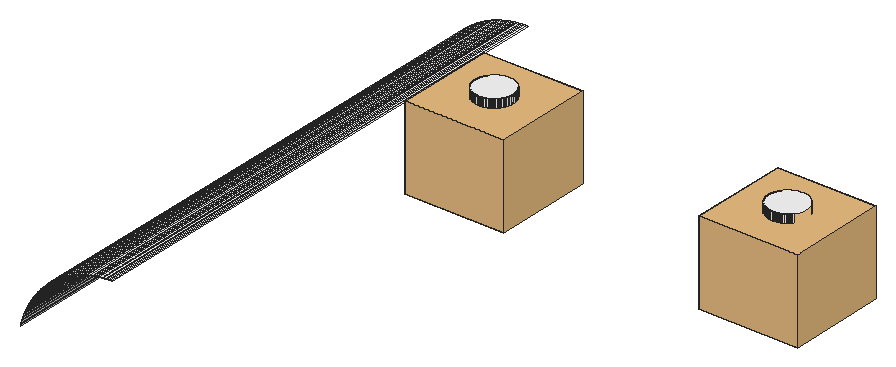
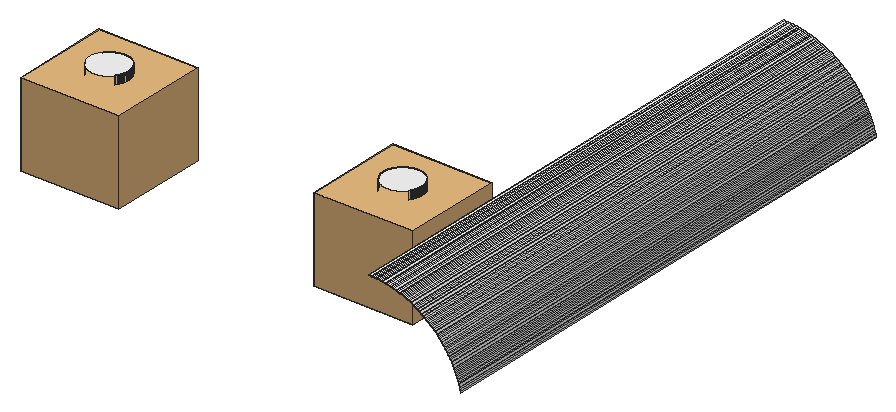
# SketchUp Ruby script. Lengths in inches.
U = 1.inch
M = Sketchup.active_model
def pt(a) = Geom::Point3d.new(a.map { |v| v * U })
def face(e, loops, mat)
  f = e.add_face(loops[0].map { |a| pt(a) })
  loops[1..].each { |l| e.add_face(l.map { |a| pt(a) }).erase! }
  f.material = f.back_material = mat if mat
  f
end
# faces: each face lists its corners as indices into pts; further lists are holes
def faces(e, pts, list, mat = nil) = list.each { |f| face(e, (f[0].is_a?(Array) ? f : [f]).map { |l| l.map { |i| pts[i] } }, mat) }
# xy, xz, yz: faces in a plane at the given z, y or x. An outline is a flat list of corners, or four numbers for a rectangle; further outlines are holes
def ring(l) = l.size == 4 ? [[l[0], l[1]], [l[2], l[1]], [l[2], l[3]], [l[0], l[3]]] : l.each_slice(2).to_a
def flat(e, list, mat, &to3) = list.each { |f| face(e, (f[0].is_a?(Array) ? f : [f]).map { |l| ring(l).map { |u, v| to3.(u, v) } }, mat) }
def xy(e, z, list, mat = nil) = flat(e, list, mat) { |x, y| [x, y, z] }
def xz(e, y, list, mat = nil) = flat(e, list, mat) { |x, z| [x, y, z] }
def yz(e, x, list, mat = nil) = flat(e, list, mat) { |y, z| [x, y, z] }
def lines(e, pts, list) = list.each { |a, b| e.add_line(pt(pts[a]), pt(pts[b])) }
# prism: a flat outline (further loops are holes) pulled along v
def prism(e, loops, v, mat = nil)
  f = face(e, loops, mat); d = Geom::Vector3d.new(v.map { |x| x * U })
  f.pushpull(f.normal.samedirection?(d) ? d.length : -d.length)
end
def box(e, o, s, mat = nil) = prism(e, [[o, [o[0] + s[0], o[1], o[2]], [o[0] + s[0], o[1] + s[1], o[2]], [o[0], o[1] + s[1], o[2]]]], [0, 0, s[2]], mat)
def at(x, y, z, deg = 0) = Geom::Transformation.translation(pt([x, y, z])) * Geom::Transformation.rotation(ORIGIN, Z_AXIS, deg.degrees)
def axes(o, x, y, z) = Geom::Transformation.new([*x, 0, *y, 0, *z, 0, *pt(o).to_a, 1])
def part(name) = M.definitions.add(name)
# library, detail: a bought-in or finely detailed component or shape, given as its bounding box
def library(name, o, s) = part(name).tap { |d| box(d.entities, o, s) }
def detail(e, o, s) = box(e.add_group.entities, o, s)
def put(e, d, t, mat = nil) = e.add_instance(d, t).tap { |i| i.material = mat if mat }
def group(e, t, mat = nil) = e.add_group.tap { |g| g.transformation = t; g.material = mat if mat }.entities
root = M.entities
M.materials.add("[Quartz Light Grey]").color = [251, 251, 252]
c1 = library("5",[-6.25,-6.25,-13.16],[15.58,15.58,13.16])
xy(root,116.99,[[59.41,189,59.61,271]],"[Quartz Light Grey]")
xy(root,117,[[59.8,189,60,271]],"[Quartz Light Grey]")
xy(root,119.5,[[68.84,250,68.76,250.01,68.6875,250.02,68.61,250.03,68.45,250.05,68.375,250.07,68.3,250.08,68.22,250.1,68.15,250.125,68.07,250.15,68,250.17,67.92,250.2,67.71,250.29,67.64,250.33,67.57,250.36,67.43,250.44,67.37,250.48,67.3,250.53,67.24,250.57,67.17,250.62,66.93,250.82,66.88,250.88,66.82,250.93,66.62,251.17,66.57,251.24,66.53,251.3,66.48,251.37,66.44,251.43,66.36,251.57,66.33,251.64,66.29,251.71,66.2,251.92,66.17,252,66.15,252.07,66.125,252.15,66.1,252.22,66.08,252.3,66.07,252.375,66.05,252.45,66.03,252.61,66.02,252.6875,66.01,252.76,66,252.84,66,253.16,66.01,253.24,66.02,253.3125,66.03,253.39,66.05,253.55,66.07,253.625,66.08,253.7,66.1,253.78,66.125,253.85,66.15,253.93,66.17,254,66.2,254.08,66.29,254.29,66.33,254.36,66.36,254.43,66.44,254.57,66.48,254.63,66.53,254.7,66.57,254.76,66.62,254.83,66.82,255.07,66.88,255.12,66.93,255.18,67.17,255.38,67.24,255.43,67.3,255.47,67.37,255.52,67.43,255.56,67.57,255.64,67.64,255.67,67.71,255.71,67.92,255.8,68,255.83,68.07,255.85,68.15,255.875,68.22,255.9,68.3,255.92,68.375,255.93,68.45,255.95,68.61,255.97,68.6875,255.98,68.76,255.99,68.84,256,69.16,256,69.24,255.99,69.3125,255.98,69.39,255.97,69.55,255.95,69.625,255.93,69.7,255.92,69.78,255.9,69.85,255.875,69.93,255.85,70,255.83,70.08,255.8,70.29,255.71,70.36,255.67,70.43,255.64,70.57,255.56,70.63,255.52,70.7,255.47,70.76,255.43,70.83,255.38,71.07,255.18,71.12,255.12,71.18,255.07,71.38,254.83,71.43,254.76,71.47,254.7,71.52,254.63,71.56,254.57,71.64,254.43,71.67,254.36,71.71,254.29,71.8,254.08,71.83,254,71.85,253.93,71.875,253.85,71.9,253.78,71.92,253.7,71.93,253.625,71.95,253.55,71.97,253.39,71.98,253.3125,71.99,253.24,72,253.16,72,252.84,71.99,252.76,71.98,252.6875,71.97,252.61,71.95,252.45,71.93,252.375,71.92,252.3,71.9,252.22,71.875,252.15,71.85,252.07,71.83,252,71.8,251.92,71.71,251.71,71.67,251.64,71.64,251.57,71.56,251.43,71.52,251.37,71.47,251.3,71.43,251.24,71.38,251.17,71.18,250.93,71.12,250.88,71.07,250.82,70.83,250.62,70.76,250.57,70.7,250.53,70.63,250.48,70.57,250.44,70.43,250.36,70.36,250.33,70.29,250.29,70.08,250.2,70,250.17,69.93,250.15,69.85,250.125,69.78,250.1,69.7,250.08,69.625,250.07,69.55,250.05,69.39,250.03,69.3125,250.02,69.24,250.01,69.16,250],[115.18,250,114.86,250.04,114.79,250.05,114.71,250.07,114.63,250.08,114.56,250.1,114.48,250.125,114.41,250.15,114.33,250.17,114.19,250.23,114.11,250.26,114.04,250.29,113.97,250.33,113.9,250.36,113.83,250.4,113.77,250.44,113.7,250.48,113.63,250.53,113.57,250.57,113.45,250.67,113.38,250.72,113.33,250.77,113.27,250.82,113.1,250.99,112.95,251.17,112.91,251.24,112.86,251.3,112.82,251.37,112.78,251.43,112.66,251.64,112.59,251.78,112.5625,251.85,112.53,251.92,112.51,252,112.48,252.07,112.46,252.15,112.4375,252.22,112.42,252.3,112.38,252.45,112.36,252.61,112.35,252.6875,112.34,252.76,112.34,252.84,112.33,252.92,112.33,253.08,112.34,253.16,112.34,253.24,112.35,253.3125,112.36,253.39,112.38,253.55,112.42,253.7,112.4375,253.78,112.46,253.85,112.48,253.93,112.51,254,112.53,254.08,112.5625,254.15,112.59,254.22,112.66,254.36,112.78,254.57,112.82,254.63,112.86,254.7,112.91,254.76,112.95,254.83,113.1,255.01,113.27,255.18,113.33,255.23,113.38,255.28,113.45,255.33,113.57,255.43,113.63,255.47,113.7,255.52,113.77,255.56,113.83,255.6,113.9,255.64,113.97,255.67,114.04,255.71,114.11,255.74,114.19,255.77,114.33,255.83,114.41,255.85,114.48,255.875,114.56,255.9,114.63,255.92,114.71,255.93,114.79,255.95,114.86,255.96,115.18,256,115.49,256,115.65,255.98,115.72,255.97,115.88,255.95,115.96,255.93,116.03,255.92,116.11,255.9,116.19,255.875,116.26,255.85,116.33,255.83,116.41,255.8,116.55,255.74,116.625,255.71,116.7,255.67,116.76,255.64,116.97,255.52,117.03,255.47,117.1,255.43,117.4,255.18,117.45,255.12,117.51,255.07,117.5625,255.01,117.61,254.95,117.71,254.83,117.76,254.76,117.81,254.7,117.85,254.63,117.89,254.57,118.01,254.36,118.13,254.08,118.16,254,118.1875,253.93,118.21,253.85,118.23,253.78,118.25,253.7,118.27,253.625,118.28,253.55,118.3,253.47,118.31,253.39,118.32,253.3125,118.32,253.24,118.33,253.16,118.33,252.84,118.32,252.76,118.32,252.6875,118.31,252.61,118.3,252.53,118.28,252.45,118.27,252.375,118.25,252.3,118.23,252.22,118.21,252.15,118.1875,252.07,118.16,252,118.13,251.92,118.01,251.64,117.89,251.43,117.85,251.37,117.81,251.3,117.76,251.24,117.71,251.17,117.61,251.05,117.5625,250.99,117.51,250.93,117.45,250.88,117.4,250.82,117.1,250.57,117.03,250.53,116.97,250.48,116.76,250.36,116.7,250.33,116.625,250.29,116.55,250.26,116.41,250.2,116.33,250.17,116.26,250.15,116.19,250.125,116.11,250.1,116.03,250.08,115.96,250.07,115.88,250.05,115.72,250.03,115.65,250.02,115.49,250]],"[Quartz Light Grey]")
xz(root,250,[[68.84,117,68.92,119.5],[68.92,117,69,119.5],[69,117,69.08,119.5],[69.08,117,69.16,119.5],[115.18,117,115.25,119.5],
  [115.25,117,115.33,119.5],[115.33,117,115.41,119.5],[115.41,117,115.49,119.5]],"[Quartz Light Grey]")
yz(root,66,[[252.84,117,252.92,119.5],[252.92,117,253,119.5],[253,117,253.08,119.5],[253.08,117,253.16,119.5]],"[Quartz Light Grey]")
yz(root,72,[[252.84,117,252.92,119.5],[252.92,117,253,119.5],[253,117,253.08,119.5],[253.08,117,253.16,119.5]],"[Quartz Light Grey]")
yz(root,112.33,[[252.92,117,253,119.5],[253,117,253.08,119.5]],"[Quartz Light Grey]")
yz(root,112.34,[[252.76,117,252.84,119.5],[253.16,117,253.24,119.5]],"[Quartz Light Grey]")
p = [[45.46,271,105.69],[45.46,189,105.69],[45.41,189,105.5],[45.41,271,105.5],[45.51,271,105.88],[45.51,189,105.88],
  [45.5625,271,106.07],[45.5625,189,106.07],[45.62,271,106.26],[45.62,189,106.26],[45.67,271,106.45],[45.67,189,106.45],
  [45.73,271,106.64],[45.73,189,106.64],[45.8,271,106.82],[45.8,189,106.82],[45.86,271,107.01],[45.86,189,107.01],
  [45.93,271,107.19],[45.93,189,107.19],[46,271,107.375],[46,189,107.375],[46.07,271,107.56],[46.07,189,107.56],
  [46.14,271,107.74],[46.14,189,107.74],[46.22,271,107.92],[46.22,189,107.92],[46.3,271,108.1],[46.3,189,108.1],
  [46.38,271,108.28],[46.38,189,108.28],[46.46,271,108.46],[46.46,189,108.46],[46.55,271,108.63],[46.55,189,108.63],
  [46.63,271,108.81],[46.63,189,108.81],[46.73,271,108.98],[46.73,189,108.98],[46.82,271,109.16],[46.82,189,109.16],
  [46.91,271,109.33],[46.91,189,109.33],[47.01,271,109.5],[47.01,189,109.5],[47.11,271,109.67],[47.11,189,109.67],
  [47.21,271,109.84],[47.21,189,109.84],[47.3125,271,110],[47.3125,189,110],[47.42,271,110.17],[47.42,189,110.17],
  [47.53,271,110.33],[47.53,189,110.33],[47.64,271,110.5],[47.64,189,110.5],[47.75,271,110.66],[47.75,189,110.66],
  [47.86,271,110.82],[47.86,189,110.82],[47.98,271,110.97],[47.98,189,110.97],[48.1,271,111.13],[48.1,189,111.13],
  [48.22,271,111.29],[48.22,189,111.29],[48.34,271,111.44],[48.34,189,111.44],[48.47,271,111.59],[48.47,189,111.59],
  [48.59,271,111.74],[48.59,189,111.74],[48.72,271,111.89],[48.72,189,111.89],[48.85,271,112.04],[48.85,189,112.04],
  [48.99,271,112.18],[48.99,189,112.18],[49.12,271,112.33],[49.12,189,112.33],[49.26,271,112.47],[49.26,189,112.47],
  [49.39,271,112.61],[49.39,189,112.61],[49.53,271,112.74],[49.53,189,112.74],[49.67,271,112.88],[49.67,189,112.88],
  [49.82,271,113.01],[49.82,189,113.01],[49.96,271,113.15],[49.96,189,113.15],[50.11,271,113.28],[50.11,189,113.28],
  [50.26,271,113.41],[50.26,189,113.41],[50.41,271,113.53],[50.41,189,113.53],[50.56,271,113.66],[50.56,189,113.66],
  [50.71,271,113.78],[50.71,189,113.78],[50.87,271,113.9],[50.87,189,113.9],[51.03,271,114.02],[51.03,189,114.02],
  [51.18,271,114.14],[51.18,189,114.14],[51.34,271,114.25],[51.34,189,114.25],[51.5,271,114.36],[51.5,189,114.36],
  [51.67,271,114.47],[51.67,189,114.47],[51.83,271,114.58],[51.83,189,114.58],[52,271,114.6875],[52,189,114.6875],
  [52.16,271,114.79],[52.16,189,114.79],[52.33,271,114.89],[52.33,189,114.89],[52.5,271,114.99],[52.5,189,114.99],
  [52.67,271,115.09],[52.67,189,115.09],[52.84,271,115.18],[52.84,189,115.18],[53.02,271,115.27],[53.02,189,115.27],
  [53.19,271,115.37],[53.19,189,115.37],[53.37,271,115.45],[53.37,189,115.45],[53.54,271,115.54],[53.54,189,115.54],
  [53.72,271,115.62],[53.72,189,115.62],[53.9,271,115.7],[53.9,189,115.7],[54.08,271,115.78],[54.08,189,115.78],
  [54.26,271,115.86],[54.26,189,115.86],[54.44,271,115.93],[54.44,189,115.93],[54.625,271,116],[54.625,189,116],
  [54.81,271,116.07],[54.81,189,116.07],[54.99,271,116.14],[54.99,189,116.14],[55.18,271,116.2],[55.18,189,116.2],
  [55.36,271,116.27],[55.36,189,116.27],[55.55,271,116.33],[55.55,189,116.33],[55.74,271,116.38],[55.74,189,116.38],
  [55.93,271,116.4375],[55.93,189,116.4375],[56.12,271,116.49],[56.12,189,116.49],[56.31,271,116.54],[56.31,189,116.54],
  [56.5,271,116.59],[56.5,189,116.59],[56.69,271,116.63],[56.69,189,116.63],[56.88,271,116.67],[56.88,189,116.67],
  [57.07,271,116.71],[57.07,189,116.71],[57.27,271,116.75],[57.27,189,116.75],[57.46,271,116.78],[57.46,189,116.78],
  [57.65,271,116.82],[57.65,189,116.82],[57.85,271,116.84],[57.85,189,116.84],[58.04,271,116.87],[58.04,189,116.87],
  [58.24,271,116.9],[58.24,189,116.9],[58.43,271,116.92],[58.43,189,116.92],[58.63,271,116.9375],[58.63,189,116.9375],
  [58.82,271,116.95],[58.82,189,116.95],[59.02,271,116.97],[59.02,189,116.97],[59.21,271,116.98],[59.21,189,116.98],
  [59.41,271,116.99],[59.41,189,116.99],[59.8,271,117],[59.8,189,117],[59.61,189,116.99],[59.61,271,116.99],
  [68.53,250.04,117],[68.45,250.05,117],[68.45,250.05,119.5],[68.53,250.04,119.5],[68.61,250.03,117],[68.61,250.03,119.5],
  [68.6875,250.02,117],[68.6875,250.02,119.5],[68.76,250.01,117],[68.76,250.01,119.5],[68.84,250,117],[68.84,250,119.5],
  [69.24,250.01,117],[69.16,250,117],[69.16,250,119.5],[69.24,250.01,119.5],[69.3125,250.02,117],[69.3125,250.02,119.5],
  [69.39,250.03,117],[69.39,250.03,119.5],[69.47,250.04,117],[69.47,250.04,119.5],[69.55,250.05,117],[69.55,250.05,119.5],
  [114.86,250.04,117],[114.79,250.05,117],[114.79,250.05,119.5],[114.86,250.04,119.5],[114.94,250.03,117],[114.94,250.03,119.5],
  [115.02,250.02,117],[115.02,250.02,119.5],[115.1,250.01,117],[115.1,250.01,119.5],[115.18,250,117],[115.18,250,119.5],
  [115.57,250.01,117],[115.49,250,117],[115.49,250,119.5],[115.57,250.01,119.5],[115.65,250.02,117],[115.65,250.02,119.5],
  [115.72,250.03,117],[115.72,250.03,119.5],[115.8,250.04,117],[115.8,250.04,119.5],[115.88,250.05,117],[115.88,250.05,119.5],
  [68.07,250.15,117],[68,250.17,117],[68,250.17,119.5],[68.07,250.15,119.5],[68.15,250.125,117],[68.15,250.125,119.5],
  [68.22,250.1,117],[68.22,250.1,119.5],[68.3,250.08,117],[68.3,250.08,119.5],[68.375,250.07,117],[68.375,250.07,119.5],
  [69.625,250.07,117],[69.625,250.07,119.5],[69.7,250.08,117],[69.7,250.08,119.5],[69.78,250.1,117],[69.78,250.1,119.5],
  [69.85,250.125,117],[69.85,250.125,119.5],[69.93,250.15,117],[69.93,250.15,119.5],[70,250.17,117],[70,250.17,119.5],
  [114.41,250.15,117],[114.33,250.17,117],[114.33,250.17,119.5],[114.41,250.15,119.5],[114.48,250.125,117],[114.48,250.125,119.5],
  [114.56,250.1,117],[114.56,250.1,119.5],[114.63,250.08,117],[114.63,250.08,119.5],[114.71,250.07,117],[114.71,250.07,119.5],
  [115.96,250.07,117],[115.96,250.07,119.5],[116.03,250.08,117],[116.03,250.08,119.5],[116.11,250.1,117],[116.11,250.1,119.5],
  [116.19,250.125,117],[116.19,250.125,119.5],[116.26,250.15,117],[116.26,250.15,119.5],[116.33,250.17,117],[116.33,250.17,119.5],
  [67.85,250.23,117],[67.78,250.26,117],[67.78,250.26,119.5],[67.85,250.23,119.5],[67.92,250.2,117],[67.92,250.2,119.5],
  [70.08,250.2,117],[70.08,250.2,119.5],[70.15,250.23,117],[70.15,250.23,119.5],[70.22,250.26,117],[70.22,250.26,119.5],
  [114.19,250.23,117],[114.11,250.26,117],[114.11,250.26,119.5],[114.19,250.23,119.5],[114.26,250.2,117],[114.26,250.2,119.5],
  [116.41,250.2,117],[116.41,250.2,119.5],[116.48,250.23,117],[116.48,250.23,119.5],[116.55,250.26,117],[116.55,250.26,119.5],
  [67.64,250.33,117],[67.57,250.36,117],[67.57,250.36,119.5],[67.64,250.33,119.5],[67.71,250.29,117],[67.71,250.29,119.5],
  [70.29,250.29,117],[70.29,250.29,119.5],[70.36,250.33,117],[70.36,250.33,119.5],[70.43,250.36,117],[70.43,250.36,119.5],
  [113.97,250.33,117],[113.9,250.36,117],[113.9,250.36,119.5],[113.97,250.33,119.5],[114.04,250.29,117],[114.04,250.29,119.5],
  [116.625,250.29,117],[116.625,250.29,119.5],[116.7,250.33,117],[116.7,250.33,119.5],[116.76,250.36,117],[116.76,250.36,119.5],
  [67.43,250.44,117],[67.37,250.48,117],[67.37,250.48,119.5],[67.43,250.44,119.5],[67.5,250.4,117],[67.5,250.4,119.5],
  [70.5,250.4,117],[70.5,250.4,119.5],[70.57,250.44,117],[70.57,250.44,119.5],[70.63,250.48,117],[70.63,250.48,119.5],
  [113.77,250.44,117],[113.7,250.48,117],[113.7,250.48,119.5],[113.77,250.44,119.5],[113.83,250.4,117],[113.83,250.4,119.5],
  [116.83,250.4,117],[116.83,250.4,119.5],[116.9,250.44,117],[116.9,250.44,119.5],[116.97,250.48,117],[116.97,250.48,119.5],
  [67.3,250.53,117],[67.24,250.57,117],[67.24,250.57,119.5],[67.3,250.53,119.5],[70.7,250.53,117],[70.7,250.53,119.5],
  [70.76,250.57,117],[70.76,250.57,119.5],[113.63,250.53,117],[113.57,250.57,117],[113.57,250.57,119.5],[113.63,250.53,119.5],
  [117.03,250.53,117],[117.03,250.53,119.5],[117.1,250.57,117],[117.1,250.57,119.5],[67.17,250.62,117],[67.11,250.67,117],
  [67.11,250.67,119.5],[67.17,250.62,119.5],[70.83,250.62,117],[70.83,250.62,119.5],[70.89,250.67,117],[70.89,250.67,119.5],
  [113.51,250.62,117],[113.45,250.67,117],[113.45,250.67,119.5],[113.51,250.62,119.5],[117.16,250.62,117],[117.16,250.62,119.5],
  [117.22,250.67,117],[117.22,250.67,119.5],[67.05,250.72,117],[66.99,250.77,117],[66.99,250.77,119.5],[67.05,250.72,119.5],
  [70.95,250.72,117],[70.95,250.72,119.5],[71.01,250.77,117],[71.01,250.77,119.5],[113.38,250.72,117],[113.33,250.77,117],
  [113.33,250.77,119.5],[113.38,250.72,119.5],[117.28,250.72,117],[117.28,250.72,119.5],[117.34,250.77,117],[117.34,250.77,119.5],
  [66.93,250.82,117],[66.88,250.88,117],[66.88,250.88,119.5],[66.93,250.82,119.5],[71.07,250.82,117],[71.07,250.82,119.5],
  [71.12,250.88,117],[71.12,250.88,119.5],[113.27,250.82,117],[113.21,250.88,117],[113.21,250.88,119.5],[113.27,250.82,119.5],
  [117.4,250.82,117],[117.4,250.82,119.5],[117.45,250.88,117],[117.45,250.88,119.5],[66.82,250.93,117],[66.77,250.99,117],
  [66.77,250.99,119.5],[66.82,250.93,119.5],[71.18,250.93,117],[71.18,250.93,119.5],[71.23,250.99,117],[71.23,250.99,119.5],
  [113.16,250.93,117],[113.1,250.99,117],[113.1,250.99,119.5],[113.16,250.93,119.5],[117.51,250.93,117],[117.51,250.93,119.5],
  [117.5625,250.99,117],[117.5625,250.99,119.5],[66.72,251.05,117],[66.72,251.05,119.5],[71.28,251.05,117],[71.28,251.05,119.5],
  [113.05,251.05,117],[113.05,251.05,119.5],[117.61,251.05,117],[117.61,251.05,119.5],[66.67,251.11,117],[66.62,251.17,117],
  [66.62,251.17,119.5],[66.67,251.11,119.5],[71.33,251.11,117],[71.33,251.11,119.5],[71.38,251.17,117],[71.38,251.17,119.5],
  [113,251.11,117],[112.95,251.17,117],[112.95,251.17,119.5],[113,251.11,119.5],[117.66,251.11,117],[117.66,251.11,119.5],
  [117.71,251.17,117],[117.71,251.17,119.5],[66.57,251.24,117],[66.53,251.3,117],[66.53,251.3,119.5],[66.57,251.24,119.5],
  [71.43,251.24,117],[71.43,251.24,119.5],[71.47,251.3,117],[71.47,251.3,119.5],[112.91,251.24,117],[112.86,251.3,117],
  [112.86,251.3,119.5],[112.91,251.24,119.5],[117.76,251.24,117],[117.76,251.24,119.5],[66.48,251.37,117],[66.48,251.37,119.5],
  [71.52,251.37,117],[71.52,251.37,119.5],[112.82,251.37,117],[112.82,251.37,119.5],[66.44,251.43,117],[66.4,251.5,117],
  [66.4,251.5,119.5],[66.44,251.43,119.5],[71.56,251.43,117],[71.56,251.43,119.5],[71.6,251.5,117],[71.6,251.5,119.5],
  [112.78,251.43,117],[112.74,251.5,117],[112.74,251.5,119.5],[112.78,251.43,119.5],[66.36,251.57,117],[66.36,251.57,119.5],
  [71.64,251.57,117],[71.64,251.57,119.5],[112.7,251.57,117],[112.7,251.57,119.5],[66.33,251.64,117],[66.29,251.71,117],
  [66.29,251.71,119.5],[66.33,251.64,119.5],[71.67,251.64,117],[71.67,251.64,119.5],[71.71,251.71,117],[71.71,251.71,119.5],
  [112.66,251.64,117],[112.625,251.71,117],[112.625,251.71,119.5],[112.66,251.64,119.5],[66.26,251.78,117],[66.26,251.78,119.5],
  [71.74,251.78,117],[71.74,251.78,119.5],[112.59,251.78,117],[112.59,251.78,119.5],[66.23,251.85,117],[66.23,251.85,119.5],
  [71.77,251.85,117],[71.77,251.85,119.5],[112.5625,251.85,117],[112.5625,251.85,119.5],[66.2,251.92,117],[66.17,252,117],
  [66.17,252,119.5],[66.2,251.92,119.5],[71.8,251.92,117],[71.8,251.92,119.5],[71.83,252,117],[71.83,252,119.5],
  [112.53,251.92,117],[112.51,252,117],[112.51,252,119.5],[112.53,251.92,119.5],[66.15,252.07,117],[66.15,252.07,119.5],
  [71.85,252.07,117],[71.85,252.07,119.5],[112.48,252.07,117],[112.48,252.07,119.5],[66.125,252.15,117],[66.1,252.22,117],
  [66.1,252.22,119.5],[66.125,252.15,119.5],[71.875,252.15,117],[71.875,252.15,119.5],[71.9,252.22,117],[71.9,252.22,119.5],
  [112.46,252.15,117],[112.4375,252.22,117],[112.4375,252.22,119.5],[112.46,252.15,119.5],[66.08,252.3,117],[66.08,252.3,119.5],
  [71.92,252.3,117],[71.92,252.3,119.5],[112.42,252.3,117],[112.42,252.3,119.5],[66.07,252.375,117],[66.07,252.375,119.5],
  [71.93,252.375,117],[71.93,252.375,119.5],[112.4,252.375,117],[112.4,252.375,119.5],[66.05,252.45,117],[66.05,252.45,119.5],
  [71.95,252.45,117],[71.95,252.45,119.5],[112.38,252.45,117],[112.38,252.45,119.5],[66.04,252.53,117],[66.03,252.61,117],
  [66.03,252.61,119.5],[66.04,252.53,119.5],[71.96,252.53,117],[71.96,252.53,119.5],[71.97,252.61,117],[71.97,252.61,119.5],
  [112.37,252.53,117],[112.36,252.61,117],[112.36,252.61,119.5],[112.37,252.53,119.5],[66.02,252.6875,117],[66.02,252.6875,119.5],
  [71.98,252.6875,117],[71.98,252.6875,119.5],[112.35,252.6875,117],[112.35,252.6875,119.5],[66.01,252.76,117],[66.01,252.76,119.5],
  [71.99,252.76,117],[71.99,252.76,119.5],[112.34,252.76,117],[112.34,252.76,119.5],[66,252.84,117],[66,252.84,119.5],
  [72,252.84,117],[72,252.84,119.5],[112.34,252.84,117],[112.33,252.92,117],[112.33,252.92,119.5],[112.34,252.84,119.5],
  [112.33,253.08,117],[112.34,253.16,117],[112.34,253.16,119.5],[112.33,253.08,119.5],[66,253.16,117],[66.01,253.24,117],
  [66.01,253.24,119.5],[66,253.16,119.5],[66.02,253.3125,117],[66.02,253.3125,119.5],[71.98,253.3125,117],[71.99,253.24,117],
  [71.99,253.24,119.5],[71.98,253.3125,119.5],[72,253.16,117],[72,253.16,119.5],[112.34,253.24,117],[112.35,253.3125,117],
  [112.35,253.3125,119.5],[112.34,253.24,119.5],[66.03,253.39,117],[66.03,253.39,119.5],[71.97,253.39,117],[71.97,253.39,119.5],
  [112.36,253.39,117],[112.36,253.39,119.5],[66.04,253.47,117],[66.04,253.47,119.5],[71.96,253.47,117],[71.96,253.47,119.5],
  [112.37,253.47,117],[112.37,253.47,119.5],[66.05,253.55,117],[66.05,253.55,119.5],[66.07,253.625,117],[66.07,253.625,119.5],
  [71.93,253.625,117],[71.95,253.55,117],[71.95,253.55,119.5],[71.93,253.625,119.5],[112.38,253.55,117],[112.38,253.55,119.5],
  [112.4,253.625,117],[112.4,253.625,119.5],[66.08,253.7,117],[66.08,253.7,119.5],[71.92,253.7,117],[71.92,253.7,119.5],
  [112.42,253.7,117],[112.42,253.7,119.5],[66.1,253.78,117],[66.1,253.78,119.5],[71.9,253.78,117],[71.9,253.78,119.5],
  [112.4375,253.78,117],[112.4375,253.78,119.5],[66.125,253.85,117],[66.125,253.85,119.5],[71.875,253.85,117],[71.875,253.85,119.5],
  [112.46,253.85,117],[112.46,253.85,119.5],[66.15,253.93,117],[66.15,253.93,119.5],[66.17,254,117],[66.17,254,119.5],
  [71.83,254,117],[71.85,253.93,117],[71.85,253.93,119.5],[71.83,254,119.5],[112.48,253.93,117],[112.48,253.93,119.5],
  [112.51,254,117],[112.51,254,119.5],[66.2,254.08,117],[66.2,254.08,119.5],[71.8,254.08,117],[71.8,254.08,119.5],
  [112.53,254.08,117],[112.53,254.08,119.5],[66.23,254.15,117],[66.23,254.15,119.5],[66.26,254.22,117],[66.26,254.22,119.5],
  [71.74,254.22,117],[71.77,254.15,117],[71.77,254.15,119.5],[71.74,254.22,119.5],[112.5625,254.15,117],[112.5625,254.15,119.5],
  [112.59,254.22,117],[112.59,254.22,119.5],[66.29,254.29,117],[66.29,254.29,119.5],[71.71,254.29,117],[71.71,254.29,119.5],
  [112.625,254.29,117],[112.625,254.29,119.5],[66.33,254.36,117],[66.33,254.36,119.5],[71.67,254.36,117],[71.67,254.36,119.5],
  [112.66,254.36,117],[112.66,254.36,119.5],[66.36,254.43,117],[66.36,254.43,119.5],[66.4,254.5,117],[66.4,254.5,119.5],
  [71.6,254.5,117],[71.64,254.43,117],[71.64,254.43,119.5],[71.6,254.5,119.5],[112.7,254.43,117],[112.7,254.43,119.5],
  [112.74,254.5,117],[112.74,254.5,119.5],[66.44,254.57,117],[66.44,254.57,119.5],[71.56,254.57,117],[71.56,254.57,119.5],
  [112.78,254.57,117],[112.78,254.57,119.5],[66.48,254.63,117],[66.48,254.63,119.5],[66.53,254.7,117],[66.53,254.7,119.5],
  [71.47,254.7,117],[71.52,254.63,117],[71.52,254.63,119.5],[71.47,254.7,119.5],[112.82,254.63,117],[112.82,254.63,119.5],
  [112.86,254.7,117],[112.86,254.7,119.5],[66.57,254.76,117],[66.57,254.76,119.5],[71.43,254.76,117],[71.43,254.76,119.5],
  [112.91,254.76,117],[112.91,254.76,119.5],[66.62,254.83,117],[66.62,254.83,119.5],[71.38,254.83,117],[71.38,254.83,119.5],
  [112.95,254.83,117],[112.95,254.83,119.5],[117.71,254.83,117],[117.76,254.76,117],[117.76,254.76,119.5],[117.71,254.83,119.5]]
faces(root,p,[[0,1,2,3],[4,5,1,0],[6,7,5,4],[8,9,7,6],[10,11,9,8],[12,13,11,10],[14,15,13,12],[16,17,15,14],
  [18,19,17,16],[20,21,19,18],[22,23,21,20],[24,25,23,22],[26,27,25,24],[28,29,27,26],[30,31,29,28],[32,33,31,30],
  [34,35,33,32],[36,37,35,34],[38,39,37,36],[40,41,39,38],[42,43,41,40],[44,45,43,42],[46,47,45,44],[48,49,47,46],
  [50,51,49,48],[52,53,51,50],[54,55,53,52],[56,57,55,54],[58,59,57,56],[60,61,59,58],[62,63,61,60],[64,65,63,62],
  [66,67,65,64],[68,69,67,66],[70,71,69,68],[72,73,71,70],[74,75,73,72],[76,77,75,74],[78,79,77,76],[80,81,79,78],
  [82,83,81,80],[84,85,83,82],[86,87,85,84],[88,89,87,86],[90,91,89,88],[92,93,91,90],[94,95,93,92],[96,97,95,94],
  [98,99,97,96],[100,101,99,98],[102,103,101,100],[104,105,103,102],[106,107,105,104],[108,109,107,106],[110,111,109,108],[112,113,111,110],
  [114,115,113,112],[116,117,115,114],[118,119,117,116],[120,121,119,118],[122,123,121,120],[124,125,123,122],[126,127,125,124],[128,129,127,126],
  [130,131,129,128],[132,133,131,130],[134,135,133,132],[136,137,135,134],[138,139,137,136],[140,141,139,138],[142,143,141,140],[144,145,143,142],
  [146,147,145,144],[148,149,147,146],[150,151,149,148],[152,153,151,150],[154,155,153,152],[156,157,155,154],[158,159,157,156],[160,161,159,158],
  [162,163,161,160],[164,165,163,162],[166,167,165,164],[168,169,167,166],[170,171,169,168],[172,173,171,170],[174,175,173,172],[176,177,175,174],
  [178,179,177,176],[180,181,179,178],[182,183,181,180],[184,185,183,182],[186,187,185,184],[188,189,187,186],[190,191,189,188],[192,193,191,190],
  [194,195,193,192],[196,197,195,194],[198,199,197,196],[200,201,202,203],[204,205,206,207],[208,204,207,209],[210,208,209,211],[212,210,211,213],
  [214,212,213,215],[216,217,218,219],[220,216,219,221],[222,220,221,223],[224,222,223,225],[226,224,225,227],[228,229,230,231],[232,228,231,233],
  [234,232,233,235],[236,234,235,237],[238,236,237,239],[240,241,242,243],[244,240,243,245],[246,244,245,247],[248,246,247,249],[250,248,249,251],
  [252,253,254,255],[256,252,255,257],[258,256,257,259],[260,258,259,261],[262,260,261,263],[205,262,263,206],[264,226,227,265],[266,264,265,267],
  [268,266,267,269],[270,268,269,271],[272,270,271,273],[274,272,273,275],[276,277,278,279],[280,276,279,281],[282,280,281,283],[284,282,283,285],
  [286,284,285,287],[229,286,287,230],[288,250,251,289],[290,288,289,291],[292,290,291,293],[294,292,293,295],[296,294,295,297],[298,296,297,299],
  [300,301,302,303],[304,300,303,305],[253,304,305,254],[306,274,275,307],[308,306,307,309],[310,308,309,311],[312,313,314,315],[316,312,315,317],
  [277,316,317,278],[318,298,299,319],[320,318,319,321],[322,320,321,323],[324,325,326,327],[328,324,327,329],[301,328,329,302],[330,310,311,331],
  [332,330,331,333],[334,332,333,335],[336,337,338,339],[340,336,339,341],[313,340,341,314],[342,322,323,343],[344,342,343,345],[346,344,345,347],
  [348,349,350,351],[352,348,351,353],[325,352,353,326],[354,334,335,355],[356,354,355,357],[358,356,357,359],[360,361,362,363],[364,360,363,365],
  [337,364,365,338],[366,346,347,367],[368,366,367,369],[370,368,369,371],[372,373,374,375],[349,372,375,350],[376,358,359,377],[378,376,377,379],
  [380,381,382,383],[361,380,383,362],[384,370,371,385],[386,384,385,387],[388,389,390,391],[373,388,391,374],[392,378,379,393],[394,392,393,395],
  [396,397,398,399],[381,396,399,382],[400,386,387,401],[402,400,401,403],[404,405,406,407],[389,404,407,390],[408,394,395,409],[410,408,409,411],
  [412,413,414,415],[397,412,415,398],[416,402,403,417],[418,416,417,419],[420,421,422,423],[405,420,423,406],[424,410,411,425],[426,424,425,427],
  [428,429,430,431],[413,428,431,414],[432,418,419,433],[434,432,433,435],[436,437,438,439],[421,436,439,422],[440,426,427,441],[442,440,441,443],
  [444,445,446,447],[429,444,447,430],[448,434,435,449],[450,448,449,451],[437,452,453,438],[454,442,443,455],[445,456,457,446],[458,450,451,459],
  [460,461,462,463],[452,460,463,453],[464,454,455,465],[466,464,465,467],[468,469,470,471],[456,468,471,457],[472,458,459,473],[474,472,473,475],
  [476,477,478,479],[461,476,479,462],[480,466,467,481],[482,480,481,483],[484,485,486,487],[469,484,487,470],[488,474,475,489],[477,490,491,478],
  [492,482,483,493],[485,494,495,486],[496,497,498,499],[490,496,499,491],[500,492,493,501],[502,500,501,503],[504,505,506,507],[494,504,507,495],
  [497,508,509,498],[510,502,503,511],[505,512,513,506],[514,515,516,517],[508,514,517,509],[518,510,511,519],[520,518,519,521],[522,523,524,525],
  [512,522,525,513],[515,526,527,516],[528,520,521,529],[523,530,531,524],[526,532,533,527],[534,528,529,535],[530,536,537,531],[538,539,540,541],
  [532,538,541,533],[542,534,535,543],[544,542,543,545],[546,547,548,549],[536,546,549,537],[539,550,551,540],[552,544,545,553],[547,554,555,548],
  [556,557,558,559],[550,556,559,551],[560,552,553,561],[562,560,561,563],[564,565,566,567],[554,564,567,555],[557,568,569,558],[570,562,563,571],
  [565,572,573,566],[568,574,575,569],[576,570,571,577],[572,578,579,573],[574,580,581,575],[582,576,577,583],[578,584,585,579],[586,587,588,589],
  [580,586,589,581],[590,582,583,591],[592,590,591,593],[594,595,596,597],[584,594,597,585],[587,598,599,588],[600,592,593,601],[595,602,603,596],
  [598,604,605,599],[606,600,601,607],[602,608,609,603],[604,610,611,605],[612,606,607,613],[614,615,616,617],[618,619,620,621],[622,623,624,625],
  [623,626,627,624],[628,629,630,631],[629,632,633,630],[634,635,636,637],[626,638,639,627],[640,628,631,641],[635,642,643,636],[638,644,645,639],
  [646,640,641,647],[642,648,649,643],[644,650,651,645],[650,652,653,651],[654,655,656,657],[655,646,647,656],[648,658,659,649],[658,660,661,659],
  [652,662,663,653],[664,654,657,665],[660,666,667,661],[662,668,669,663],[670,664,665,671],[666,672,673,667],[668,674,675,669],[676,670,671,677],
  [672,678,679,673],[674,680,681,675],[680,682,683,681],[684,685,686,687],[685,676,677,686],[678,688,689,679],[688,690,691,689],[682,692,693,683],
  [694,684,687,695],[690,696,697,691],[692,698,699,693],[698,700,701,699],[702,703,704,705],[703,694,695,704],[696,706,707,697],[706,708,709,707],
  [700,710,711,701],[712,702,705,713],[708,714,715,709],[710,716,717,711],[718,712,713,719],[714,720,721,715],[716,722,723,717],[722,724,725,723],
  [726,727,728,729],[727,718,719,728],[720,730,731,721],[730,732,733,731],[724,734,735,725],[736,726,729,737],[732,738,739,733],[734,740,741,735],
  [740,742,743,741],[744,745,746,747],[745,736,737,746],[738,748,749,739],[748,750,751,749],[742,752,753,743],[754,744,747,755],[750,756,757,751],
  [752,758,759,753],[760,754,755,761],[756,762,763,757],[764,765,766,767]],"[Quartz Light Grey]")
put(root,c1,at(67.46,251.46,118.25),"[Quartz Light Grey]")
put(root,c1,at(113.8,251.46,118.25),"[Quartz Light Grey]")
